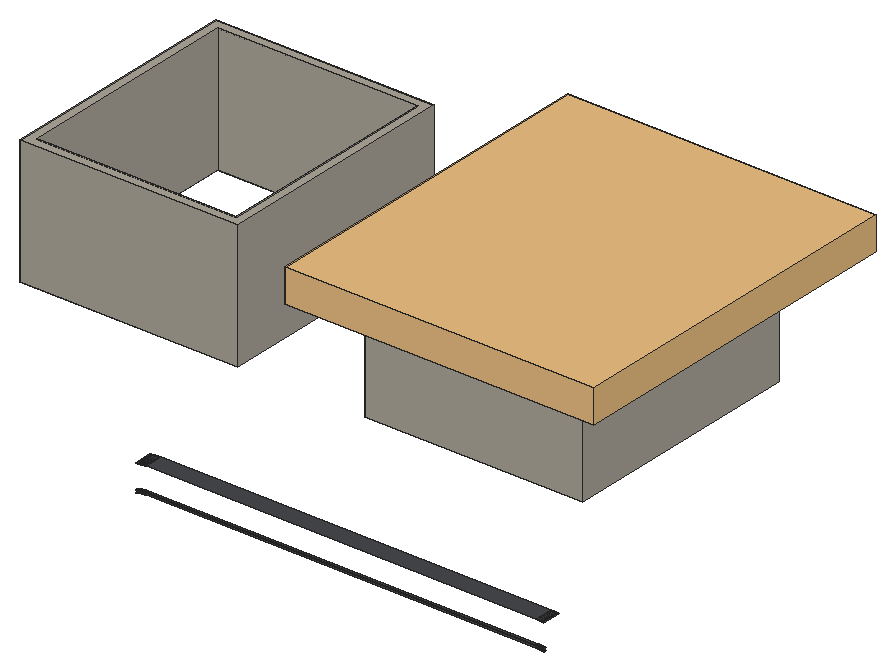
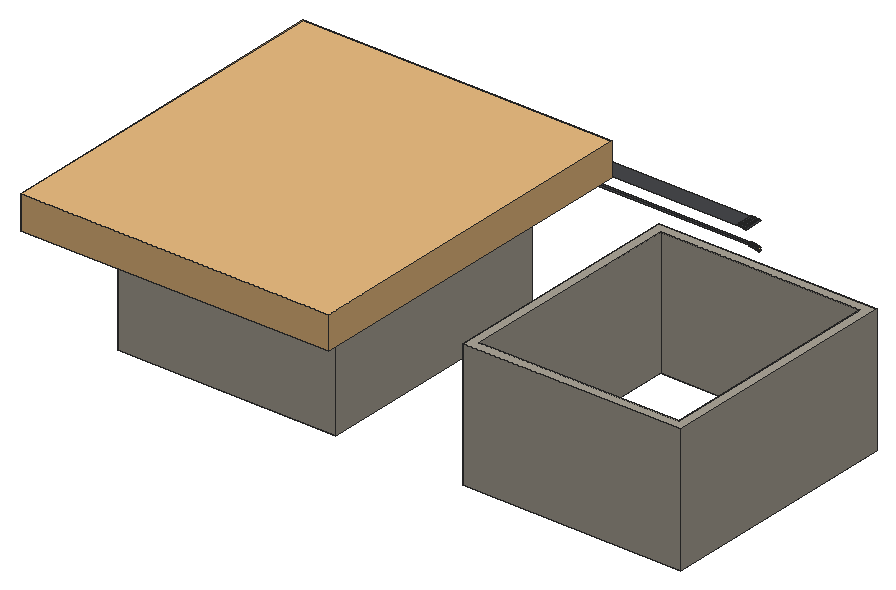
# SketchUp Ruby script. Lengths in inches.
U = 1.inch
M = Sketchup.active_model
def pt(a) = Geom::Point3d.new(a.map { |v| v * U })
def face(e, loops, mat)
  f = e.add_face(loops[0].map { |a| pt(a) })
  loops[1..].each { |l| e.add_face(l.map { |a| pt(a) }).erase! }
  f.material = f.back_material = mat if mat
  f
end
# faces: each face lists its corners as indices into pts; further lists are holes
def faces(e, pts, list, mat = nil) = list.each { |f| face(e, (f[0].is_a?(Array) ? f : [f]).map { |l| l.map { |i| pts[i] } }, mat) }
# xy, xz, yz: faces in a plane at the given z, y or x. An outline is a flat list of corners, or four numbers for a rectangle; further outlines are holes
def ring(l) = l.size == 4 ? [[l[0], l[1]], [l[2], l[1]], [l[2], l[3]], [l[0], l[3]]] : l.each_slice(2).to_a
def flat(e, list, mat, &to3) = list.each { |f| face(e, (f[0].is_a?(Array) ? f : [f]).map { |l| ring(l).map { |u, v| to3.(u, v) } }, mat) }
def xy(e, z, list, mat = nil) = flat(e, list, mat) { |x, y| [x, y, z] }
def xz(e, y, list, mat = nil) = flat(e, list, mat) { |x, z| [x, y, z] }
def yz(e, x, list, mat = nil) = flat(e, list, mat) { |y, z| [x, y, z] }
def lines(e, pts, list) = list.each { |a, b| e.add_line(pt(pts[a]), pt(pts[b])) }
# prism: a flat outline (further loops are holes) pulled along v
def prism(e, loops, v, mat = nil)
  f = face(e, loops, mat); d = Geom::Vector3d.new(v.map { |x| x * U })
  f.pushpull(f.normal.samedirection?(d) ? d.length : -d.length)
end
def box(e, o, s, mat = nil) = prism(e, [[o, [o[0] + s[0], o[1], o[2]], [o[0] + s[0], o[1] + s[1], o[2]], [o[0], o[1] + s[1], o[2]]]], [0, 0, s[2]], mat)
def at(x, y, z, deg = 0) = Geom::Transformation.translation(pt([x, y, z])) * Geom::Transformation.rotation(ORIGIN, Z_AXIS, deg.degrees)
def axes(o, x, y, z) = Geom::Transformation.new([*x, 0, *y, 0, *z, 0, *pt(o).to_a, 1])
def part(name) = M.definitions.add(name)
# library, detail: a bought-in or finely detailed component or shape, given as its bounding box
def library(name, o, s) = part(name).tap { |d| box(d.entities, o, s) }
def detail(e, o, s) = box(e.add_group.entities, o, s)
def put(e, d, t, mat = nil) = e.add_instance(d, t).tap { |i| i.material = mat if mat }
def group(e, t, mat = nil) = e.add_group.tap { |g| g.transformation = t; g.material = mat if mat }.entities
root = M.entities
M.materials.add("1432 AP 8245 TAR ROAD").color = [71, 72, 75]
M.materials.add("Generic").color = [172, 166, 153]
M.materials.add("Outer Light").color = [251, 217, 152]
c1 = library("2",[-24,-36,-9.91],[204,234,21.91])
xy(root,579.78,[[278.25,95.37,278.4,96.87],[537.6,95.37,537.75,96.87]],"1432 AP 8245 TAR ROAD")
xy(root,579.78,[[278.25,95.37,278.4,96.87],[537.6,95.37,537.75,96.87]],"Outer Light")
xy(root,579.79,[[278.55,95.37,278.7,96.87],[278.7,95.37,278.85,96.87],[278.85,95.37,279,96.87],[279,95.37,537,96.87],[537,95.37,537.15,96.87],
  [537.15,95.37,537.3,96.87],[537.3,95.37,537.45,96.87]],"1432 AP 8245 TAR ROAD")
xy(root,579.79,[[278.55,95.37,278.7,96.87],[278.7,95.37,278.85,96.87],[278.85,95.37,279,96.87],[279,95.37,537,96.87],[537,95.37,537.15,96.87],
  [537.15,95.37,537.3,96.87],[537.3,95.37,537.45,96.87]],"Outer Light")
xy(root,581.28,[[278.2,95.37,278.36,96.87],[537.64,95.37,537.8,96.87]],"1432 AP 8245 TAR ROAD")
xy(root,581.28,[[278.2,95.37,278.36,96.87],[537.64,95.37,537.8,96.87]],"Outer Light")
xy(root,581.29,[[278.52,95.37,278.68,96.87],[278.68,95.37,278.84,96.87],[278.84,95.37,279,96.87],[279,95.37,537,96.87],[537,95.37,537.16,96.87],
  [537.16,95.37,537.32,96.87],[537.32,95.37,537.48,96.87]],"1432 AP 8245 TAR ROAD")
xy(root,581.29,[[278.52,95.37,278.68,96.87],[278.68,95.37,278.84,96.87],[278.84,95.37,279,96.87],[279,95.37,537,96.87],[537,95.37,537.16,96.87],
  [537.16,95.37,537.32,96.87],[537.32,95.37,537.48,96.87]],"Outer Light")
xy(root,596.79,[[278.43,95.37,278.72,107.37],[278.72,95.37,279,107.37],[279,95.37,537,107.37],[537,95.37,537.28,107.37],[537.28,95.37,537.57,107.37]],"1432 AP 8245 TAR ROAD")
p = [[272.01,95.37,578.46],[272.14,95.37,578.51],[272.14,96.87,578.51],[272.01,96.87,578.46],[272.01,96.87,578.46],[272.14,96.87,578.51],
  [272.14,95.37,578.51],[272.01,95.37,578.46],[272.28,95.37,578.57],[272.28,96.87,578.57],[272.28,96.87,578.57],[272.28,95.37,578.57],
  [272.42,95.37,578.62],[272.42,96.87,578.62],[272.42,96.87,578.62],[272.42,95.37,578.62],[272.5625,95.37,578.67],[272.5625,96.87,578.67],
  [272.5625,96.87,578.67],[272.5625,95.37,578.67],[272.7,95.37,578.72],[272.7,96.87,578.72],[272.7,96.87,578.72],[272.7,95.37,578.72],
  [272.85,95.37,578.77],[272.85,96.87,578.77],[272.85,96.87,578.77],[272.85,95.37,578.77],[272.99,95.37,578.82],[272.99,96.87,578.82],
  [272.99,96.87,578.82],[272.99,95.37,578.82],[273.13,95.37,578.86],[273.13,96.87,578.86],[273.13,96.87,578.86],[273.13,95.37,578.86],
  [273.27,95.37,578.91],[273.27,96.87,578.91],[273.27,96.87,578.91],[273.27,95.37,578.91],[273.41,95.37,578.95],[273.41,96.87,578.95],
  [273.41,96.87,578.95],[273.41,95.37,578.95],[273.56,95.37,579],[273.56,96.87,579],[273.56,96.87,579],[273.56,95.37,579],
  [273.7,95.37,579.04],[273.7,96.87,579.04],[273.7,96.87,579.04],[273.7,95.37,579.04],[273.84,95.37,579.08],[273.84,96.87,579.08],
  [273.84,96.87,579.08],[273.84,95.37,579.08],[273.99,95.37,579.12],[273.99,96.87,579.12],[273.99,96.87,579.12],[273.99,95.37,579.12],
  [274.13,95.37,579.16],[274.13,96.87,579.16],[274.13,96.87,579.16],[274.13,95.37,579.16],[541.87,95.37,579.16],[542.01,95.37,579.12],
  [542.01,96.87,579.12],[541.87,96.87,579.16],[541.87,96.87,579.16],[542.01,96.87,579.12],[542.01,95.37,579.12],[541.87,95.37,579.16],
  [274.27,95.37,579.2],[274.27,96.87,579.2],[274.27,96.87,579.2],[274.27,95.37,579.2],[274.42,95.37,579.23],[274.42,96.87,579.23],
  [274.42,96.87,579.23],[274.42,95.37,579.23],[274.56,95.37,579.27],[274.56,96.87,579.27],[274.56,96.87,579.27],[274.56,95.37,579.27],
  [541.44,95.37,579.27],[541.58,95.37,579.23],[541.58,96.87,579.23],[541.44,96.87,579.27],[541.44,96.87,579.27],[541.58,96.87,579.23],
  [541.58,95.37,579.23],[541.44,95.37,579.27],[541.73,95.37,579.2],[541.73,96.87,579.2],[541.73,96.87,579.2],[541.73,95.37,579.2],
  [274.71,95.37,579.3],[274.71,96.87,579.3],[274.71,96.87,579.3],[274.71,95.37,579.3],[274.86,95.37,579.33],[274.86,96.87,579.33],
  [274.86,96.87,579.33],[274.86,95.37,579.33],[275,95.37,579.37],[275,96.87,579.37],[275,96.87,579.37],[275,95.37,579.37],
  [541,95.37,579.37],[541.14,95.37,579.33],[541.14,96.87,579.33],[541,96.87,579.37],[541,96.87,579.37],[541.14,96.87,579.33],
  [541.14,95.37,579.33],[541,95.37,579.37],[541.29,95.37,579.3],[541.29,96.87,579.3],[541.29,96.87,579.3],[541.29,95.37,579.3],
  [275.15,95.37,579.4],[275.15,96.87,579.4],[275.15,96.87,579.4],[275.15,95.37,579.4],[275.29,95.37,579.43],[275.29,96.87,579.43],
  [275.29,96.87,579.43],[275.29,95.37,579.43],[275.44,95.37,579.46],[275.44,96.87,579.46],[275.44,96.87,579.46],[275.44,95.37,579.46],
  [540.56,95.37,579.46],[540.71,95.37,579.43],[540.71,96.87,579.43],[540.56,96.87,579.46],[540.56,96.87,579.46],[540.71,96.87,579.43],
  [540.71,95.37,579.43],[540.56,95.37,579.46],[540.85,95.37,579.4],[540.85,96.87,579.4],[540.85,96.87,579.4],[540.85,95.37,579.4],
  [275.59,95.37,579.48],[275.59,96.87,579.48],[275.59,96.87,579.48],[275.59,95.37,579.48],[275.73,95.37,579.51],[275.73,96.87,579.51],
  [275.73,96.87,579.51],[275.73,95.37,579.51],[275.88,95.37,579.53],[275.88,96.87,579.53],[275.88,96.87,579.53],[275.88,95.37,579.53],
  [276.03,95.37,579.56],[276.03,96.87,579.56],[276.03,96.87,579.56],[276.03,95.37,579.56],[539.97,95.37,579.56],[540.12,95.37,579.53],
  [540.12,96.87,579.53],[539.97,96.87,579.56],[539.97,96.87,579.56],[540.12,96.87,579.53],[540.12,95.37,579.53],[539.97,95.37,579.56],
  [540.27,95.37,579.51],[540.27,96.87,579.51],[540.27,96.87,579.51],[540.27,95.37,579.51],[540.41,95.37,579.48],[540.41,96.87,579.48],
  [540.41,96.87,579.48],[540.41,95.37,579.48],[276.18,95.37,579.58],[276.18,96.87,579.58],[276.18,96.87,579.58],[276.18,95.37,579.58],
  [276.32,95.37,579.6],[276.32,96.87,579.6],[276.32,96.87,579.6],[276.32,95.37,579.6],[276.47,95.37,579.62],[276.47,96.87,579.62],
  [276.47,96.87,579.62],[276.47,95.37,579.62],[276.62,95.37,579.64],[276.62,96.87,579.64],[276.62,96.87,579.64],[276.62,95.37,579.64],
  [276.77,95.37,579.66],[276.77,96.87,579.66],[276.77,96.87,579.66],[276.77,95.37,579.66],[539.23,95.37,579.66],[539.38,95.37,579.64],
  [539.38,96.87,579.64],[539.23,96.87,579.66],[539.23,96.87,579.66],[539.38,96.87,579.64],[539.38,95.37,579.64],[539.23,95.37,579.66],
  [539.53,95.37,579.62],[539.53,96.87,579.62],[539.53,96.87,579.62],[539.53,95.37,579.62],[539.68,95.37,579.6],[539.68,96.87,579.6],
  [539.68,96.87,579.6],[539.68,95.37,579.6],[539.82,95.37,579.58],[539.82,96.87,579.58],[539.82,96.87,579.58],[539.82,95.37,579.58],
  [276.92,95.37,579.68],[276.92,96.87,579.68],[276.92,96.87,579.68],[276.92,95.37,579.68],[277.0625,95.37,579.69],[277.0625,96.87,579.69],
  [277.0625,96.87,579.69],[277.0625,95.37,579.69],[277.21,95.37,579.71],[277.21,96.87,579.71],[277.21,96.87,579.71],[277.21,95.37,579.71],
  [277.36,95.37,579.72],[277.36,96.87,579.72],[277.36,96.87,579.72],[277.36,95.37,579.72],[277.51,95.37,579.73],[277.51,96.87,579.73],
  [277.51,96.87,579.73],[277.51,95.37,579.73],[277.66,95.37,579.74],[277.66,96.87,579.74],[277.66,96.87,579.74],[277.66,95.37,579.74],
  [277.81,95.37,579.75],[277.81,96.87,579.75],[277.81,96.87,579.75],[277.81,95.37,579.75],[538.19,95.37,579.75],[538.34,95.37,579.74],
  [538.34,96.87,579.74],[538.19,96.87,579.75],[538.19,96.87,579.75],[538.34,96.87,579.74],[538.34,95.37,579.74],[538.19,95.37,579.75],
  [538.49,95.37,579.73],[538.49,96.87,579.73],[538.49,96.87,579.73],[538.49,95.37,579.73],[538.64,95.37,579.72],[538.64,96.87,579.72],
  [538.64,96.87,579.72],[538.64,95.37,579.72],[538.79,95.37,579.71],[538.79,96.87,579.71],[538.79,96.87,579.71],[538.79,95.37,579.71],
  [538.9375,95.37,579.69],[538.9375,96.87,579.69],[538.9375,96.87,579.69],[538.9375,95.37,579.69],[539.08,95.37,579.68],[539.08,96.87,579.68],
  [539.08,96.87,579.68],[539.08,95.37,579.68],[277.96,95.37,579.76],[277.96,96.87,579.76],[277.96,96.87,579.76],[277.96,95.37,579.76],
  [278.1,95.37,579.77],[278.1,96.87,579.77],[278.1,96.87,579.77],[278.1,95.37,579.77],[278.25,95.37,579.78],[278.25,96.87,579.78],
  [278.25,96.87,579.78],[278.25,95.37,579.78],[278.4,95.37,579.78],[278.55,95.37,579.79],[278.55,96.87,579.79],[278.4,96.87,579.78],
  [278.4,96.87,579.78],[278.55,96.87,579.79],[278.55,95.37,579.79],[278.4,95.37,579.78],[537.45,95.37,579.79],[537.6,95.37,579.78],
  [537.6,96.87,579.78],[537.45,96.87,579.79],[537.45,96.87,579.79],[537.6,96.87,579.78],[537.6,95.37,579.78],[537.45,95.37,579.79],
  [537.75,95.37,579.78],[537.9,95.37,579.77],[537.9,96.87,579.77],[537.75,96.87,579.78],[537.75,96.87,579.78],[537.9,96.87,579.77],
  [537.9,95.37,579.77],[537.75,95.37,579.78],[538.04,95.37,579.76],[538.04,96.87,579.76],[538.04,96.87,579.76],[538.04,95.37,579.76],
  [272.06,96.87,580.08],[271.9,96.87,580.02],[271.9,95.37,580.02],[272.06,95.37,580.08],[272.21,96.87,580.13],[272.21,95.37,580.13],
  [272.21,95.37,580.13],[272.06,95.37,580.08],[272.06,96.87,580.08],[272.21,96.87,580.13],[272.36,96.87,580.1875],[272.36,95.37,580.1875],
  [272.36,95.37,580.1875],[272.36,96.87,580.1875],[272.51,96.87,580.24],[272.51,95.37,580.24],[272.51,95.37,580.24],[272.51,96.87,580.24],
  [272.67,96.87,580.29],[272.67,95.37,580.29],[272.67,95.37,580.29],[272.67,96.87,580.29],[272.82,96.87,580.34],[272.82,95.37,580.34],
  [272.82,95.37,580.34],[272.82,96.87,580.34],[272.97,96.87,580.39],[272.97,95.37,580.39],[272.97,95.37,580.39],[272.97,96.87,580.39],
  [273.125,96.87,580.43],[273.125,95.37,580.43],[273.125,95.37,580.43],[273.125,96.87,580.43],[273.28,96.87,580.48],[273.28,95.37,580.48],
  [273.28,95.37,580.48],[273.28,96.87,580.48],[273.44,96.87,580.52],[273.44,95.37,580.52],[273.44,95.37,580.52],[273.44,96.87,580.52],
  [273.59,96.87,580.57],[273.59,95.37,580.57],[273.59,95.37,580.57],[273.59,96.87,580.57],[273.75,96.87,580.61],[273.75,95.37,580.61],
  [273.75,95.37,580.61],[273.75,96.87,580.61],[273.9,96.87,580.65],[273.9,95.37,580.65],[273.9,95.37,580.65],[273.9,96.87,580.65],
  [274.06,96.87,580.6875],[274.06,95.37,580.6875],[274.06,95.37,580.6875],[274.06,96.87,580.6875],[274.21,96.87,580.73],[274.21,95.37,580.73],
  [274.21,95.37,580.73],[274.21,96.87,580.73],[274.37,96.87,580.76],[274.37,95.37,580.76],[274.37,95.37,580.76],[274.37,96.87,580.76],
  [541.79,96.87,580.73],[541.63,96.87,580.76],[541.63,95.37,580.76],[541.79,95.37,580.73],[541.79,95.37,580.73],[541.63,95.37,580.76],
  [541.63,96.87,580.76],[541.79,96.87,580.73],[541.94,96.87,580.6875],[541.94,95.37,580.6875],[541.94,95.37,580.6875],[541.94,96.87,580.6875],
  [274.53,96.87,580.8],[274.53,95.37,580.8],[274.53,95.37,580.8],[274.53,96.87,580.8],[274.69,96.87,580.83],[274.69,95.37,580.83],
  [274.69,95.37,580.83],[274.69,96.87,580.83],[274.84,96.87,580.87],[274.84,95.37,580.87],[274.84,95.37,580.87],[274.84,96.87,580.87],
  [541.31,96.87,580.83],[541.16,96.87,580.87],[541.16,95.37,580.87],[541.31,95.37,580.83],[541.31,95.37,580.83],[541.16,95.37,580.87],
  [541.16,96.87,580.87],[541.31,96.87,580.83],[541.47,96.87,580.8],[541.47,95.37,580.8],[541.47,95.37,580.8],[541.47,96.87,580.8],
  [275,96.87,580.9],[275,95.37,580.9],[275,95.37,580.9],[275,96.87,580.9],[275.16,96.87,580.93],[275.16,95.37,580.93],
  [275.16,95.37,580.93],[275.16,96.87,580.93],[275.32,96.87,580.96],[275.32,95.37,580.96],[275.32,95.37,580.96],[275.32,96.87,580.96],
  [540.84,96.87,580.93],[540.68,96.87,580.96],[540.68,95.37,580.96],[540.84,95.37,580.93],[540.84,95.37,580.93],[540.68,95.37,580.96],
  [540.68,96.87,580.96],[540.84,96.87,580.93],[541,96.87,580.9],[541,95.37,580.9],[541,95.37,580.9],[541,96.87,580.9],
  [275.48,96.87,580.99],[275.48,95.37,580.99],[275.48,95.37,580.99],[275.48,96.87,580.99],[275.63,96.87,581.01],[275.63,95.37,581.01],
  [275.63,95.37,581.01],[275.63,96.87,581.01],[275.79,96.87,581.04],[275.79,95.37,581.04],[275.79,95.37,581.04],[275.79,96.87,581.04],
  [275.95,96.87,581.0625],[275.95,95.37,581.0625],[275.95,95.37,581.0625],[275.95,96.87,581.0625],[540.21,96.87,581.04],[540.05,96.87,581.0625],
  [540.05,95.37,581.0625],[540.21,95.37,581.04],[540.21,95.37,581.04],[540.05,95.37,581.0625],[540.05,96.87,581.0625],[540.21,96.87,581.04],
  [540.37,96.87,581.01],[540.37,95.37,581.01],[540.37,95.37,581.01],[540.37,96.87,581.01],[540.52,96.87,580.99],[540.52,95.37,580.99],
  [540.52,95.37,580.99],[540.52,96.87,580.99],[276.11,96.87,581.09],[276.11,95.37,581.09],[276.11,95.37,581.09],[276.11,96.87,581.09],
  [276.27,96.87,581.11],[276.27,95.37,581.11],[276.27,95.37,581.11],[276.27,96.87,581.11],[276.43,96.87,581.13],[276.43,95.37,581.13],
  [276.43,95.37,581.13],[276.43,96.87,581.13],[276.59,96.87,581.15],[276.59,95.37,581.15],[276.59,95.37,581.15],[276.59,96.87,581.15],
  [276.75,96.87,581.17],[276.75,95.37,581.17],[276.75,95.37,581.17],[276.75,96.87,581.17],[539.41,96.87,581.15],[539.25,96.87,581.17],
  [539.25,95.37,581.17],[539.41,95.37,581.15],[539.41,95.37,581.15],[539.25,95.37,581.17],[539.25,96.87,581.17],[539.41,96.87,581.15],
  [539.57,96.87,581.13],[539.57,95.37,581.13],[539.57,95.37,581.13],[539.57,96.87,581.13],[539.73,96.87,581.11],[539.73,95.37,581.11],
  [539.73,95.37,581.11],[539.73,96.87,581.11],[539.89,96.87,581.09],[539.89,95.37,581.09],[539.89,95.37,581.09],[539.89,96.87,581.09],
  [276.91,96.87,581.19],[276.91,95.37,581.19],[276.91,95.37,581.19],[276.91,96.87,581.19],[277.07,96.87,581.2],[277.07,95.37,581.2],
  [277.07,95.37,581.2],[277.07,96.87,581.2],[277.23,96.87,581.22],[277.23,95.37,581.22],[277.23,95.37,581.22],[277.23,96.87,581.22],
  [277.39,96.87,581.23],[277.39,95.37,581.23],[277.39,95.37,581.23],[277.39,96.87,581.23],[277.55,96.87,581.24],[277.55,95.37,581.24],
  [277.55,95.37,581.24],[277.55,96.87,581.24],[277.71,96.87,581.25],[277.71,95.37,581.25],[277.71,95.37,581.25],[277.71,96.87,581.25],
  [538.45,96.87,581.24],[538.29,96.87,581.25],[538.29,95.37,581.25],[538.45,95.37,581.24],[538.45,95.37,581.24],[538.29,95.37,581.25],
  [538.29,96.87,581.25],[538.45,96.87,581.24],[538.61,96.87,581.23],[538.61,95.37,581.23],[538.61,95.37,581.23],[538.61,96.87,581.23],
  [538.77,96.87,581.22],[538.77,95.37,581.22],[538.77,95.37,581.22],[538.77,96.87,581.22],[538.93,96.87,581.2],[538.93,95.37,581.2],
  [538.93,95.37,581.2],[538.93,96.87,581.2],[539.09,96.87,581.19],[539.09,95.37,581.19],[539.09,95.37,581.19],[539.09,96.87,581.19],
  [277.875,96.87,581.26],[277.875,95.37,581.26],[277.875,95.37,581.26],[277.875,96.87,581.26],[278.03,96.87,581.27],[278.03,95.37,581.27],
  [278.03,95.37,581.27],[278.03,96.87,581.27],[278.2,96.87,581.28],[278.2,95.37,581.28],[278.2,95.37,581.28],[278.2,96.87,581.28],
  [278.52,96.87,581.29],[278.36,96.87,581.28],[278.36,95.37,581.28],[278.52,95.37,581.29],[278.52,95.37,581.29],[278.36,95.37,581.28],
  [278.36,96.87,581.28],[278.52,96.87,581.29],[537.64,96.87,581.28],[537.48,96.87,581.29],[537.48,95.37,581.29],[537.64,95.37,581.28],
  [537.64,95.37,581.28],[537.48,95.37,581.29],[537.48,96.87,581.29],[537.64,96.87,581.28],[537.97,96.87,581.27],[537.8,96.87,581.28],
  [537.8,95.37,581.28],[537.97,95.37,581.27],[537.97,95.37,581.27],[537.8,95.37,581.28],[537.8,96.87,581.28],[537.97,96.87,581.27],
  [538.125,96.87,581.26],[538.125,95.37,581.26],[538.125,95.37,581.26],[538.125,96.87,581.26],[272.25,107.37,596.15],[271.98,107.37,596.1],
  [271.98,95.37,596.1],[272.25,95.37,596.15],[272.53,107.37,596.21],[272.53,95.37,596.21],[272.8125,107.37,596.26],[272.8125,95.37,596.26],
  [273.09,107.37,596.3],[273.09,95.37,596.3],[273.37,107.37,596.35],[273.37,95.37,596.35],[273.65,107.37,596.39],[273.65,95.37,596.39],
  [273.93,107.37,596.43],[273.93,95.37,596.43],[274.21,107.37,596.47],[274.21,95.37,596.47],[542.07,107.37,596.43],[541.79,107.37,596.47],
  [541.79,95.37,596.47],[542.07,95.37,596.43],[274.49,107.37,596.51],[274.49,95.37,596.51],[274.77,107.37,596.54],[274.77,95.37,596.54],
  [275.05,107.37,596.57],[275.05,95.37,596.57],[541.23,107.37,596.54],[540.95,107.37,596.57],[540.95,95.37,596.57],[541.23,95.37,596.54],
  [541.51,107.37,596.51],[541.51,95.37,596.51],[275.33,107.37,596.6],[275.33,95.37,596.6],[275.61,107.37,596.63],[275.61,95.37,596.63],
  [275.89,107.37,596.66],[275.89,95.37,596.66],[540.39,107.37,596.63],[540.11,107.37,596.66],[540.11,95.37,596.66],[540.39,95.37,596.63],
  [540.67,107.37,596.6],[540.67,95.37,596.6],[276.18,107.37,596.68],[276.18,95.37,596.68],[276.46,107.37,596.7],[276.46,95.37,596.7],
  [276.74,107.37,596.72],[276.74,95.37,596.72],[277.02,107.37,596.74],[277.02,95.37,596.74],[277.3,107.37,596.75],[277.3,95.37,596.75],
  [538.98,107.37,596.74],[538.7,107.37,596.75],[538.7,95.37,596.75],[538.98,95.37,596.74],[539.26,107.37,596.72],[539.26,95.37,596.72],
  [539.54,107.37,596.7],[539.54,95.37,596.7],[539.82,107.37,596.68],[539.82,95.37,596.68],[277.59,107.37,596.76],[277.59,95.37,596.76],
  [277.87,107.37,596.77],[277.87,95.37,596.77],[278.15,107.37,596.78],[278.15,95.37,596.78],[278.43,107.37,596.79],[278.43,95.37,596.79],
  [537.85,107.37,596.78],[537.57,107.37,596.79],[537.57,95.37,596.79],[537.85,95.37,596.78],[538.13,107.37,596.77],[538.13,95.37,596.77],
  [538.41,107.37,596.76],[538.41,95.37,596.76]]
faces(root,p,[[0,1,2,3],[1,8,9,2],[8,12,13,9],[12,16,17,13],[16,20,21,17],[20,24,25,21],[24,28,29,25],[28,32,33,29],
  [32,36,37,33],[36,40,41,37],[40,44,45,41],[44,48,49,45],[48,52,53,49],[52,56,57,53],[56,60,61,57],[64,65,66,67],
  [60,72,73,61],[72,76,77,73],[76,80,81,77],[84,85,86,87],[85,92,93,86],[92,64,67,93],[80,96,97,81],[96,100,101,97],
  [100,104,105,101],[108,109,110,111],[109,116,117,110],[116,84,87,117],[104,120,121,105],[120,124,125,121],[124,128,129,125],[132,133,134,135],
  [133,140,141,134],[140,108,111,141],[128,144,145,129],[144,148,149,145],[148,152,153,149],[152,156,157,153],[160,161,162,163],[161,168,169,162],
  [168,172,173,169],[172,132,135,173],[156,176,177,157],[176,180,181,177],[180,184,185,181],[184,188,189,185],[188,192,193,189],[196,197,198,199],
  [197,204,205,198],[204,208,209,205],[208,212,213,209],[212,160,163,213],[192,216,217,193],[216,220,221,217],[220,224,225,221],[224,228,229,225],
  [228,232,233,229],[232,236,237,233],[236,240,241,237],[244,245,246,247],[245,252,253,246],[252,256,257,253],[256,260,261,257],[260,264,265,261],
  [264,268,269,265],[268,196,199,269],[240,272,273,241],[272,276,277,273],[276,280,281,277],[284,285,286,287],[292,293,294,295],[300,301,302,303],
  [301,308,309,302],[308,244,247,309],[318,319,320,321],[324,318,321,325],[328,324,325,329],[332,328,329,333],[336,332,333,337],[340,336,337,341],
  [344,340,341,345],[348,344,345,349],[352,348,349,353],[356,352,353,357],[360,356,357,361],[364,360,361,365],[368,364,365,369],[372,368,369,373],
  [376,372,373,377],[382,383,384,385],[388,382,385,389],[392,376,377,393],[396,392,393,397],[400,396,397,401],[406,407,408,409],[412,406,409,413],
  [383,412,413,384],[416,400,401,417],[420,416,417,421],[424,420,421,425],[430,431,432,433],[436,430,433,437],[407,436,437,408],[440,424,425,441],
  [444,440,441,445],[448,444,445,449],[452,448,449,453],[458,459,460,461],[464,458,461,465],[468,464,465,469],[431,468,469,432],[472,452,453,473],
  [476,472,473,477],[480,476,477,481],[484,480,481,485],[488,484,485,489],[494,495,496,497],[500,494,497,501],[504,500,501,505],[508,504,505,509],
  [459,508,509,460],[512,488,489,513],[516,512,513,517],[520,516,517,521],[524,520,521,525],[528,524,525,529],[532,528,529,533],[538,539,540,541],
  [544,538,541,545],[548,544,545,549],[552,548,549,553],[556,552,553,557],[495,556,557,496],[560,532,533,561],[564,560,561,565],[568,564,565,569],
  [574,575,576,577],[582,583,584,585],[590,591,592,593],[596,590,593,597],[539,596,597,540],[598,599,600,601],[602,598,601,603],[604,602,603,605],
  [606,604,605,607],[608,606,607,609],[610,608,609,611],[612,610,611,613],[614,612,613,615],[616,617,618,619],[620,614,615,621],[622,620,621,623],
  [624,622,623,625],[626,627,628,629],[630,626,629,631],[617,630,631,618],[632,624,625,633],[634,632,633,635],[636,634,635,637],[638,639,640,641],
  [642,638,641,643],[627,642,643,628],[644,636,637,645],[646,644,645,647],[648,646,647,649],[650,648,649,651],[652,650,651,653],[654,655,656,657],
  [658,654,657,659],[660,658,659,661],[662,660,661,663],[639,662,663,640],[664,652,653,665],[666,664,665,667],[668,666,667,669],[670,668,669,671],
  [672,673,674,675],[676,672,675,677],[678,676,677,679],[655,678,679,656]],"1432 AP 8245 TAR ROAD")
faces(root,p,[[4,5,6,7],[5,10,11,6],[10,14,15,11],[14,18,19,15],[18,22,23,19],[22,26,27,23],[26,30,31,27],[30,34,35,31],
  [34,38,39,35],[38,42,43,39],[42,46,47,43],[46,50,51,47],[50,54,55,51],[54,58,59,55],[58,62,63,59],[68,69,70,71],
  [62,74,75,63],[74,78,79,75],[78,82,83,79],[88,89,90,91],[89,94,95,90],[94,68,71,95],[82,98,99,83],[98,102,103,99],
  [102,106,107,103],[112,113,114,115],[113,118,119,114],[118,88,91,119],[106,122,123,107],[122,126,127,123],[126,130,131,127],[136,137,138,139],
  [137,142,143,138],[142,112,115,143],[130,146,147,131],[146,150,151,147],[150,154,155,151],[154,158,159,155],[164,165,166,167],[165,170,171,166],
  [170,174,175,171],[174,136,139,175],[158,178,179,159],[178,182,183,179],[182,186,187,183],[186,190,191,187],[190,194,195,191],[200,201,202,203],
  [201,206,207,202],[206,210,211,207],[210,214,215,211],[214,164,167,215],[194,218,219,195],[218,222,223,219],[222,226,227,223],[226,230,231,227],
  [230,234,235,231],[234,238,239,235],[238,242,243,239],[248,249,250,251],[249,254,255,250],[254,258,259,255],[258,262,263,259],[262,266,267,263],
  [266,270,271,267],[270,200,203,271],[242,274,275,243],[274,278,279,275],[278,282,283,279],[288,289,290,291],[296,297,298,299],[304,305,306,307],
  [305,310,311,306],[310,248,251,311],[312,313,314,315],[316,312,315,317],[322,316,317,323],[326,322,323,327],[330,326,327,331],[334,330,331,335],
  [338,334,335,339],[342,338,339,343],[346,342,343,347],[350,346,347,351],[354,350,351,355],[358,354,355,359],[362,358,359,363],[366,362,363,367],
  [370,366,367,371],[374,370,371,375],[378,379,380,381],[386,378,381,387],[390,374,375,391],[394,390,391,395],[398,394,395,399],[402,403,404,405],
  [410,402,405,411],[379,410,411,380],[414,398,399,415],[418,414,415,419],[422,418,419,423],[426,427,428,429],[434,426,429,435],[403,434,435,404],
  [438,422,423,439],[442,438,439,443],[446,442,443,447],[450,446,447,451],[454,455,456,457],[462,454,457,463],[466,462,463,467],[427,466,467,428],
  [470,450,451,471],[474,470,471,475],[478,474,475,479],[482,478,479,483],[486,482,483,487],[490,491,492,493],[498,490,493,499],[502,498,499,503],
  [506,502,503,507],[455,506,507,456],[510,486,487,511],[514,510,511,515],[518,514,515,519],[522,518,519,523],[526,522,523,527],[530,526,527,531],
  [534,535,536,537],[542,534,537,543],[546,542,543,547],[550,546,547,551],[554,550,551,555],[491,554,555,492],[558,530,531,559],[562,558,559,563],
  [566,562,563,567],[570,571,572,573],[578,579,580,581],[586,587,588,589],[594,586,589,595],[535,594,595,536]],"Outer Light")
g1 = group(root,at(90,227.37,581.79),"Generic")
prism(g1,[[[0,0,0],[0,162,0],[144,162,0],[144,0,0]],[[6,156,0],[6,6,0],[138,6,0],[138,156,0]]],[0,0,84])
prism(g1,[[[228,162,0],[372,162,0],[372,0,0],[228,0,0]],[[234,156,0],[234,6,0],[366,6,0],[366,156,0]]],[0,0,84])
put(root,c1,at(318,227.37,665.79))
